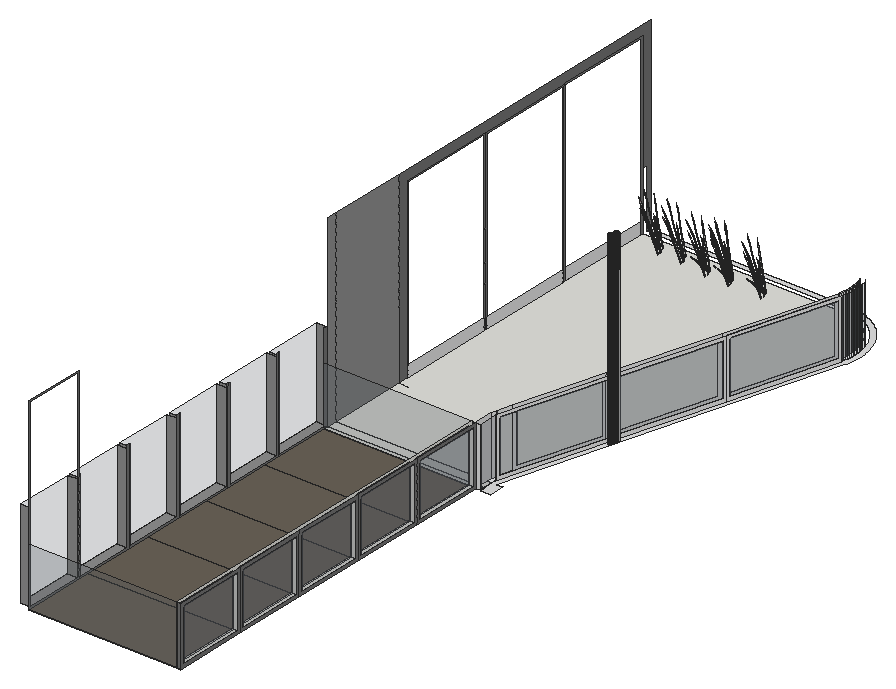
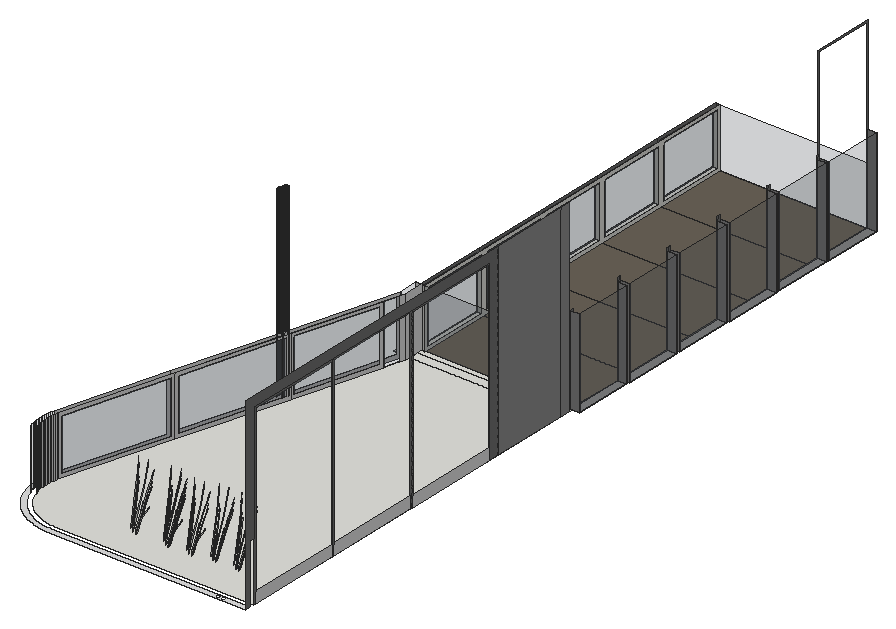
# SketchUp Ruby script. Lengths in inches.
U = 1.inch
M = Sketchup.active_model
def pt(a) = Geom::Point3d.new(a.map { |v| v * U })
def face(e, loops, mat)
  f = e.add_face(loops[0].map { |a| pt(a) })
  loops[1..].each { |l| e.add_face(l.map { |a| pt(a) }).erase! }
  f.material = f.back_material = mat if mat
  f
end
# faces: each face lists its corners as indices into pts; further lists are holes
def faces(e, pts, list, mat = nil) = list.each { |f| face(e, (f[0].is_a?(Array) ? f : [f]).map { |l| l.map { |i| pts[i] } }, mat) }
# xy, xz, yz: faces in a plane at the given z, y or x. An outline is a flat list of corners, or four numbers for a rectangle; further outlines are holes
def ring(l) = l.size == 4 ? [[l[0], l[1]], [l[2], l[1]], [l[2], l[3]], [l[0], l[3]]] : l.each_slice(2).to_a
def flat(e, list, mat, &to3) = list.each { |f| face(e, (f[0].is_a?(Array) ? f : [f]).map { |l| ring(l).map { |u, v| to3.(u, v) } }, mat) }
def xy(e, z, list, mat = nil) = flat(e, list, mat) { |x, y| [x, y, z] }
def xz(e, y, list, mat = nil) = flat(e, list, mat) { |x, z| [x, y, z] }
def yz(e, x, list, mat = nil) = flat(e, list, mat) { |y, z| [x, y, z] }
def lines(e, pts, list) = list.each { |a, b| e.add_line(pt(pts[a]), pt(pts[b])) }
# prism: a flat outline (further loops are holes) pulled along v
def prism(e, loops, v, mat = nil)
  f = face(e, loops, mat); d = Geom::Vector3d.new(v.map { |x| x * U })
  f.pushpull(f.normal.samedirection?(d) ? d.length : -d.length)
end
def box(e, o, s, mat = nil) = prism(e, [[o, [o[0] + s[0], o[1], o[2]], [o[0] + s[0], o[1] + s[1], o[2]], [o[0], o[1] + s[1], o[2]]]], [0, 0, s[2]], mat)
def at(x, y, z, deg = 0) = Geom::Transformation.translation(pt([x, y, z])) * Geom::Transformation.rotation(ORIGIN, Z_AXIS, deg.degrees)
def axes(o, x, y, z) = Geom::Transformation.new([*x, 0, *y, 0, *z, 0, *pt(o).to_a, 1])
def part(name) = M.definitions.add(name)
# library, detail: a bought-in or finely detailed component or shape, given as its bounding box
def library(name, o, s) = part(name).tap { |d| box(d.entities, o, s) }
def detail(e, o, s) = box(e.add_group.entities, o, s)
def put(e, d, t, mat = nil) = e.add_instance(d, t).tap { |i| i.material = mat if mat }
def group(e, t, mat = nil) = e.add_group.tap { |g| g.transformation = t; g.material = mat if mat }.entities
root = M.entities
M.materials.add("Glass_Basic_01").color = [105, 113, 122]
M.materials["Glass_Basic_01"].alpha = 0.25
M.materials.add("LightPink_Translucent").color = [144, 107, 117]
M.materials["LightPink_Translucent"].alpha = 0.75
M.materials.add("M01_Silver_Fog").color = [224, 224, 224]
M.materials.add("M04_Stone_Frost").color = [142, 142, 142]
M.materials.add("M06_Steel_Smoke").color = [114, 114, 114]
M.materials.add("Plaster_04_1K").color = [106, 98, 87]
c1 = part("blade")
p = [[2.15,0.21,22],[0,0.17,0],[0.09,0.45,0],[2.18,0.31,22],[2.29,0.31,22],[0.38,0.45,0],
  [2.48,0.24,33],[2.49,0.24,33],[2.48,0.22,33]]
faces(c1.entities,p,[[0,1,2,3],[4,5,2,3],[6,3,4,7],[8,0,3,6]])
c2 = part("seeds")
p = [[0.3,-0.1,1.38],[-0.01,-0.03,1.59],[-0.01,-0.03,0.03],[0.14,-0.07,-0.07],[0.29,-0.03,3],[0.15,0.01,3.11]]
faces(c2.entities,p,[[0,1,2,3],[1,0,4,5]],"LightPink_Translucent")
c3 = part("blade with seeds")
put(c3.entities,c1,at(0,0,0))
put(c3.entities,c2,axes([2.4,0.25,30.99],[1.5799,-0.05474,1.17369],[-0.12525,1.92788,0.29478],[-0.07173,-0.02425,1.56792]))
xy(root,648,[[210,231,302.38,234],[302.38,231,305.51,234],[305.51,231,306,234],[210,234,302.38,240],[302.38,234,305.51,240],
  [210,240,302.38,240,302.38,243,303.26,246,306,255.36,321.22,307.35,340.07,371.78,359.17,437.01,359.4,437.91,359.63,439,359.83,440.1,359.98,441.21,360.09,442.32,360.16,443.43,360.1875,444.55,360.17,445.67,360.11,446.78,360.01,447.89,359.87,449,359.68,450.1,359.45,451.2,359.18,452.28,358.875,453.35,358.52,454.41,358.13,455.46,357.7,456.49,357.23,457.5,356.73,458.5,356.18,459.47,355.6,460.43,354.98,461.36,354.33,462.26,353.64,463.14,352.92,464,352.17,464.83,351.39,465.62,350.58,466.39,349.74,467.125,348.87,467.83,347.97,468.5,347.05,469.13,346.11,469.73,345.15,470.29,344.16,470.82,343.16,471.3,342.13,471.75,341.09,472.16,340.04,472.53,338.97,472.86,337.89,473.15,336.8,473.4,335.71,473.6,334.6,473.77,333.49,473.89,332.38,473.97,331.45,474,210,474]])
xy(root,648,[[[306,231,312,231,312,240,307.76,240,364.95,435.42,365.24,436.52,365.52,437.84,365.76,439.16,365.94,440.5,366.07,441.84,366.16,443.18,366.1875,444.52,366.17,445.87,366.1,447.21,365.98,448.55,365.8,449.89,365.58,451.21,365.3,452.53,364.98,453.84,364.61,455.13,364.18,456.41,363.71,457.67,363.2,458.91,362.63,460.13,362.02,461.33,361.36,462.5,360.69,463.59,360.66,463.65,359.92,464.77,359.13,465.86,358.3,466.92,357.4375,467.95,357.39,468,356.53,468.95,355.59,469.91,354.61,470.83,353.6,471.72,352.55,472.5625,351.47,473.37,350.37,474.13,349.23,474.85,348.07,475.53,346.88,476.16,345.67,476.75,344.44,477.29,343.1875,477.79,341.92,478.23,340.63,478.63,339.33,478.98,338.02,479.28,336.7,479.52,335.37,479.72,334.03,479.87,332.69,479.96,331.55,480,210,480,210,477,331.5,477,332.53,476.97,333.76,476.88,334.99,476.74,336.2,476.5625,337.41,476.34,338.61,476.0625,339.8,475.75,340.98,475.38,342.14,474.97,343.29,474.52,344.41,474.03,345.52,473.49,346.61,472.91,347.67,472.29,348.71,471.63,349.72,470.93,350.71,470.19,351.67,469.42,352.59,468.61,353.49,467.76,354.35,466.89,355.17,465.98,355.18,465.98,355.97,465.03,356.73,464.0625,357.45,463.0625,358.13,462.04,358.13,462.03,358.77,460.99,359.37,459.91,359.93,458.82,360.45,457.7,360.92,456.5625,361.35,455.41,361.74,454.24,362.08,453.06,362.38,451.86,362.63,450.66,362.83,449.44,362.99,448.22,363.1,447,363.17,445.77,363.1875,444.54,363.16,443.31,363.08,442.08,362.96,440.85,362.79,439.63,362.58,438.42,362.32,437.22,362.06,436.22,343.2,371.78,324.34,307.35,305.51,243,305.51,234,306,234],[228.34,477.03,228.25,477.04,228.17,477.06,228.08,477.08,228,477.11,227.91,477.14,227.84,477.18,227.76,477.22,227.68,477.27,227.54,477.37,227.48,477.43,227.42,477.5,227.36,477.56,227.3125,477.64,227.26,477.71,227.18,477.87,227.15,477.95,227.125,478.03,227.1,478.12,227.09,478.2,227.07,478.29,227.07,478.55,227.08,478.64,227.1,478.73,227.12,478.8125,227.15,478.9,227.18,478.98,227.22,479.06,227.26,479.13,227.31,479.21,227.41,479.35,227.47,479.41,227.61,479.53,227.75,479.63,227.91,479.71,228.07,479.77,228.16,479.79,228.24,479.81,228.33,479.82,228.42,479.82,228.51,479.83,228.59,479.82,228.68,479.81,228.77,479.79,228.85,479.77,228.9375,479.74,229.02,479.71,229.1,479.68,229.18,479.63,229.25,479.59,229.32,479.53,229.39,479.48,229.45,479.42,229.51,479.35,229.57,479.29,229.62,479.22,229.67,479.14,229.71,479.07,229.75,478.99,229.78,478.9,229.81,478.82,229.83,478.74,229.85,478.65,229.86,478.5625,229.87,478.47,229.87,478.39,229.85,478.21,229.83,478.125,229.8125,478.04,229.79,477.96,229.75,477.875,229.72,477.79,229.67,477.72,229.63,477.64,229.58,477.57,229.52,477.5,229.46,477.4375,229.4,477.38,229.33,477.32,229.26,477.27,229.18,477.22,229.11,477.18,229.03,477.14,228.95,477.11,228.86,477.08,228.78,477.06,228.69,477.04,228.6,477.03],[225.03,477.03,224.94,477.04,224.85,477.06,224.77,477.08,224.68,477.11,224.6,477.14,224.52,477.18,224.45,477.22,224.37,477.27,224.23,477.37,224.17,477.43,224.11,477.5,224.05,477.56,224,477.64,223.95,477.71,223.87,477.87,223.84,477.95,223.8125,478.03,223.77,478.2,223.76,478.29,223.76,478.55,223.77,478.64,223.79,478.73,223.81,478.8125,223.84,478.9,223.87,478.98,223.91,479.06,223.95,479.13,223.99,479.21,224.05,479.28,224.1,479.35,224.16,479.41,224.23,479.47,224.29,479.53,224.36,479.58,224.4375,479.63,224.52,479.67,224.6,479.71,224.76,479.77,224.85,479.79,224.93,479.81,225.02,479.82,225.11,479.82,225.19,479.83,225.37,479.81,225.46,479.79,225.54,479.77,225.71,479.71,225.79,479.68,225.86,479.63,225.9375,479.59,226.01,479.53,226.08,479.48,226.14,479.42,226.2,479.35,226.26,479.29,226.3125,479.22,226.36,479.14,226.4,479.07,226.4375,478.99,226.47,478.9,226.5,478.82,226.52,478.74,226.54,478.65,226.55,478.5625,226.55,478.3,226.54,478.21,226.5,478.04,226.47,477.96,226.44,477.875,226.4,477.79,226.36,477.72,226.32,477.64,226.26,477.57,226.21,477.5,226.15,477.4375,226.08,477.38,226.02,477.32,225.95,477.27,225.87,477.22,225.71,477.14,225.55,477.08,225.46,477.06,225.38,477.04,225.29,477.03],[325.27,304.17,325.18,304.18,325.09,304.1875,325.01,304.2,324.92,304.23,324.84,304.25,324.6,304.37,324.39,304.52,324.32,304.58,324.26,304.65,324.11,304.86,324.03,305.02,324,305.1,323.97,305.1875,323.95,305.27,323.9375,305.36,323.93,305.44,323.92,305.53,323.92,305.62,323.93,305.71,323.9375,305.8,323.96,305.88,323.98,305.97,324,306.05,324.12,306.29,324.27,306.5,324.33,306.56,324.4,306.625,324.47,306.68,324.61,306.78,324.77,306.86,324.85,306.89,324.9375,306.92,325.02,306.9375,325.11,306.95,325.2,306.96,325.28,306.97,325.37,306.97,325.55,306.95,325.63,306.93,325.72,306.91,325.88,306.85,325.96,306.8125,326.04,306.77,326.18,306.67,326.25,306.61,326.31,306.55,326.375,306.49,326.43,306.42,326.53,306.28,326.61,306.12,326.64,306.04,326.67,305.95,326.6875,305.87,326.7,305.78,326.71,305.69,326.72,305.61,326.72,305.52,326.7,305.34,326.68,305.26,326.66,305.17,326.6,305.01,326.5625,304.93,326.52,304.85,326.42,304.71,326.3,304.57,326.24,304.51,326.03,304.36,325.87,304.28,325.79,304.25,325.7,304.22,325.62,304.2,325.53,304.1875,325.44,304.17],[326.2,307.35,326.02,307.37,325.9375,307.38,325.85,307.41,325.77,307.43,325.6875,307.47,325.61,307.5,325.53,307.55,325.32,307.7,325.26,307.76,325.14,307.9,325.04,308.04,324.96,308.2,324.93,308.28,324.9,308.37,324.88,308.45,324.87,308.54,324.85,308.71,324.85,308.8,324.87,308.98,324.89,309.0625,324.91,309.15,324.9375,309.23,324.97,309.3125,325.01,309.39,325.05,309.47,325.2,309.68,325.27,309.74,325.33,309.8,325.4,309.86,325.54,309.96,325.7,310.04,325.78,310.07,325.87,310.1,325.95,310.12,326.04,310.13,326.21,310.15,326.3,310.15,326.48,310.13,326.5625,310.11,326.65,310.09,326.73,310.0625,326.8125,310.03,326.89,309.99,326.97,309.95,327.11,309.85,327.25,309.73,327.31,309.67,327.46,309.46,327.54,309.3,327.57,309.22,327.6,309.13,327.62,309.05,327.63,308.96,327.65,308.79,327.65,308.7,327.63,308.52,327.61,308.4375,327.59,308.35,327.56,308.27,327.53,308.1875,327.49,308.11,327.45,308.03,327.4,307.96,327.35,307.88,327.3,307.82,327.17,307.69,326.96,307.54,326.8,307.46,326.72,307.43,326.63,307.4,326.55,307.38,326.46,307.36,326.375,307.35]]],"M01_Silver_Fog")
xy(root,648,[[300,6,303,51],[300,51,303,96],[300,96,303,141],[300,141,303,186],[300,186,303,231]],"M06_Steel_Smoke")
xy(root,648,[[210,6,300,51],[210,51,300,96],[210,96,300,141],[210,141,300,186],[210,186,300,231]],"Plaster_04_1K")
xy(root,649,[[204,7,210,43],[204,45,210,81],[204,83,210,119],[204,121,210,157],[204,159,210,195],
  [204,197,210,233]],"M04_Stone_Frost")
xy(root,650,[[300,8,303,49],[300,53,303,94],[300,98,303,139],[300,143,303,184],[300,188,303,229]])
xz(root,6,[[210,648,300,684]],"Glass_Basic_01")
xz(root,6,[[300,648,303,684]],"M06_Steel_Smoke")
xz(root,7,[[204,649,210,703]],"M04_Stone_Frost")
xz(root,8,[[300,650,303,682]])
xz(root,43,[[204,649,210,703]],"M04_Stone_Frost")
xz(root,45,[[204,649,210,703]],"M04_Stone_Frost")
xz(root,49,[[300,650,303,682]])
xz(root,53,[[300,650,303,682]])
xz(root,81,[[204,649,210,703]],"M04_Stone_Frost")
xz(root,83,[[204,649,210,703]],"M04_Stone_Frost")
xz(root,94,[[300,650,303,682]])
xz(root,98,[[300,650,303,682]])
xz(root,119,[[204,649,210,703]],"M04_Stone_Frost")
xz(root,121,[[204,649,210,703]],"M04_Stone_Frost")
xz(root,139,[[300,650,303,682]])
xz(root,143,[[300,650,303,682]])
xz(root,157,[[204,649,210,703]],"M04_Stone_Frost")
xz(root,159,[[204,649,210,703]],"M04_Stone_Frost")
xz(root,184,[[300,650,303,682]])
xz(root,188,[[300,650,303,682]])
xz(root,195,[[204,649,210,703]],"M04_Stone_Frost")
xz(root,197,[[204,649,210,703]],"M04_Stone_Frost")
xz(root,229,[[300,650,303,682]])
xz(root,231,[[300,648,302.38,684]])
xz(root,231,[[210,648,300,684]],"Glass_Basic_01")
xz(root,231,[[302.38,648,303,684],[303,648,305.51,684]],"M01_Silver_Fog")
xz(root,233,[[204,649,210,703]],"M04_Stone_Frost")
xz(root,304.17,[[325.27,648,325.36,762],[325.36,648,325.44,762]],"M01_Silver_Fog")
xz(root,306.97,[[325.28,648,325.37,762]],"M01_Silver_Fog")
xz(root,307.35,[[326.2,648,326.29,762],[326.29,648,326.375,762]],"M01_Silver_Fog")
xz(root,310.15,[[326.21,648,326.3,762]],"M01_Silver_Fog")
yz(root,204,[[7,649,43,703],[45,649,81,703],[83,649,119,703],[121,649,157,703],[159,649,195,703],
  [197,649,233,703]],"Glass_Basic_01")
yz(root,210,[[295,648,353,655],[355,648,413,655],[415,648,473,655]],"M01_Silver_Fog")
yz(root,210,[[234,648,240,762],[240,648,288,762]],"M04_Stone_Frost")
yz(root,210,[[6,648,44,648,44,705,43,705,43,649,7,649,7,761,43,761,43,705,44,705,44,762,6,762],[44,648,82,648,82,705,81,705,81,649,45,649,45,705,44,705],[82,648,120,648,120,705,119,705,119,649,83,649,83,705,82,705],[120,648,158,648,158,705,157,705,157,649,121,649,121,705,120,705],[158,648,196,648,196,705,195,705,195,649,159,649,159,705,158,705],
  [196,648,231,648,231,649,197,649,197,705,196,705],[288,648,294,648,294,756,474,756,474,684,477,684,477,648,480,648,480,762,288,762],[294,648,295,648,295,755,353,755,353,648,354,648,354,756,294,756],[354,648,355,648,355,755,413,755,413,648,414,648,414,756,354,756],[414,648,415,648,415,755,473,755,473,648,474,648,474,756,414,756],
  [231,649,233,703]],"M06_Steel_Smoke")
yz(root,300,[[[6,648,231,684],[8,650,49,682],[143,650,184,682],[188,650,229,682],[53,650,94,682],[98,650,139,682]]])
yz(root,300,[[8,650,49,682],[53,650,94,682],[98,650,139,682],[143,650,184,682],[188,650,229,682]],"Glass_Basic_01")
yz(root,302.38,[[231,648,243,684]],"M01_Silver_Fog")
yz(root,303,[[8,650,49,682],[53,650,94,682],[98,650,139,682],[143,650,184,682],[188,650,229,682]],"Glass_Basic_01")
yz(root,303,[[[6,648,51,684],[8,650,49,682]],[[51,648,96,684],[53,650,94,682]],[[96,648,141,684],[98,650,139,682]],[[141,648,186,684],[143,650,184,682]],[[186,648,231,684],[188,650,229,682]]],"M06_Steel_Smoke")
yz(root,305.51,[[231,648,243,684]],"Glass_Basic_01")
yz(root,323.92,[[305.53,648,305.62,762]],"M01_Silver_Fog")
yz(root,324.85,[[308.71,648,308.8,762]],"M01_Silver_Fog")
yz(root,326.72,[[305.52,648,305.61,762]],"M01_Silver_Fog")
yz(root,327.65,[[308.7,648,308.79,762]],"M01_Silver_Fog")
p = [[302.38,243,684],[303.26,246,684],[303.26,246,648],[302.38,243,648],[305.51,243,648],[324.34,307.35,648],
  [324.34,307.35,684],[305.51,243,684],[323.78,305.43,682],[323.78,305.43,650],[306.07,244.92,650],[306.07,244.92,682],
  [306,255.36,684],[306,255.36,648],[321.22,307.35,684],[321.22,307.35,648],[320.65,305.43,682],[306.5625,257.28,682],
  [306.5625,257.28,650],[320.65,305.43,650],[324.84,304.25,648],[324.92,304.23,648],[324.92,304.23,762],[324.84,304.25,762],
  [325.01,304.2,648],[325.01,304.2,762],[325.09,304.1875,648],[325.09,304.1875,762],[325.18,304.18,648],[325.18,304.18,762],
  [325.27,304.17,648],[325.27,304.17,762],[325.44,304.17,648],[325.53,304.1875,648],[325.53,304.1875,762],[325.44,304.17,762],
  [325.62,304.2,648],[325.62,304.2,762],[325.7,304.22,648],[325.7,304.22,762],[325.79,304.25,648],[325.79,304.25,762],
  [325.87,304.28,648],[325.87,304.28,762],[324.6,304.37,648],[324.68,304.33,648],[324.68,304.33,762],[324.6,304.37,762],
  [324.76,304.29,648],[324.76,304.29,762],[325.95,304.32,648],[325.95,304.32,762],[326.03,304.36,648],[326.03,304.36,762],
  [324.53,304.42,648],[324.53,304.42,762],[324.46,304.47,648],[324.46,304.47,762],[326.1,304.41,648],[326.1,304.41,762],
  [326.17,304.46,648],[326.17,304.46,762],[324.32,304.58,648],[324.39,304.52,648],[324.39,304.52,762],[324.32,304.58,762],
  [326.24,304.51,648],[326.24,304.51,762],[326.3,304.57,648],[326.3,304.57,762],[324.21,304.72,648],[324.26,304.65,648],
  [324.26,304.65,762],[324.21,304.72,762],[326.36,304.64,648],[326.36,304.64,762],[326.42,304.71,648],[326.42,304.71,762],
  [324.16,304.79,648],[324.16,304.79,762],[326.47,304.78,648],[326.47,304.78,762],[324.11,304.86,648],[324.11,304.86,762],
  [326.52,304.85,648],[326.52,304.85,762],[324.03,305.02,648],[324.07,304.94,648],[324.07,304.94,762],[324.03,305.02,762],
  [326.5625,304.93,648],[326.5625,304.93,762],[326.6,305.01,648],[326.6,305.01,762],[324,305.1,648],[324,305.1,762],
  [326.63,305.09,648],[326.63,305.09,762],[323.97,305.1875,648],[323.97,305.1875,762],[326.66,305.17,648],[326.66,305.17,762],
  [323.95,305.27,648],[323.95,305.27,762],[326.68,305.26,648],[326.68,305.26,762],[323.9375,305.36,648],[323.9375,305.36,762],
  [326.7,305.34,648],[326.7,305.34,762],[326.71,305.43,648],[326.71,305.43,762],[323.93,305.44,648],[323.93,305.44,762],
  [323.92,305.53,648],[323.92,305.53,762],[326.72,305.52,648],[326.72,305.52,762],[323.93,305.71,648],[323.92,305.62,648],
  [323.92,305.62,762],[323.93,305.71,762],[326.72,305.61,648],[326.71,305.69,648],[326.71,305.69,762],[326.72,305.61,762],
  [323.9375,305.8,648],[323.9375,305.8,762],[326.7,305.78,648],[326.7,305.78,762],[323.96,305.88,648],[323.96,305.88,762],
  [326.6875,305.87,648],[326.6875,305.87,762],[323.98,305.97,648],[323.98,305.97,762],[326.67,305.95,648],[326.67,305.95,762],
  [324,306.05,648],[324,306.05,762],[326.64,306.04,648],[326.64,306.04,762],[326.61,306.12,648],[326.61,306.12,762],
  [324.04,306.13,648],[324.04,306.13,762],[324.08,306.21,648],[324.08,306.21,762],[326.57,306.2,648],[326.57,306.2,762],
  [324.12,306.29,648],[324.12,306.29,762],[326.53,306.28,648],[326.53,306.28,762],[324.17,306.36,648],[324.17,306.36,762],
  [326.48,306.35,648],[326.48,306.35,762],[324.22,306.43,648],[324.22,306.43,762],[324.27,306.5,648],[324.27,306.5,762],
  [326.43,306.42,648],[326.43,306.42,762],[326.375,306.49,648],[326.375,306.49,762],[324.33,306.56,648],[324.33,306.56,762],
  [326.31,306.55,648],[326.31,306.55,762],[324.4,306.625,648],[324.4,306.625,762],[324.47,306.68,648],[324.47,306.68,762],
  [326.25,306.61,648],[326.18,306.67,648],[326.18,306.67,762],[326.25,306.61,762],[324.54,306.73,648],[324.54,306.73,762],
  [324.61,306.78,648],[324.61,306.78,762],[326.11,306.72,648],[326.04,306.77,648],[326.04,306.77,762],[326.11,306.72,762],
  [324.69,306.82,648],[324.69,306.82,762],[324.77,306.86,648],[324.77,306.86,762],[325.96,306.8125,648],[325.88,306.85,648],
  [325.88,306.85,762],[325.96,306.8125,762],[324.85,306.89,648],[324.85,306.89,762],[324.9375,306.92,648],[324.9375,306.92,762],
  [325.02,306.9375,648],[325.02,306.9375,762],[325.11,306.95,648],[325.11,306.95,762],[325.63,306.93,648],[325.55,306.95,648],
  [325.55,306.95,762],[325.63,306.93,762],[325.72,306.91,648],[325.72,306.91,762],[325.8,306.88,648],[325.8,306.88,762],
  [325.2,306.96,648],[325.2,306.96,762],[325.28,306.97,648],[325.28,306.97,762],[325.46,306.96,648],[325.37,306.97,648],
  [325.37,306.97,762],[325.46,306.96,762],[340.07,371.78,684],[340.07,371.78,648],[339.51,369.86,650],[339.51,369.86,682],
  [321.78,309.27,682],[321.78,309.27,650],[343.2,371.78,684],[343.2,371.78,648],[324.9,309.27,650],[324.9,309.27,682],
  [342.64,369.86,682],[342.64,369.86,650],[326.11,307.36,648],[326.2,307.35,648],[326.2,307.35,762],[326.11,307.36,762],
  [325.6875,307.47,648],[325.77,307.43,648],[325.77,307.43,762],[325.6875,307.47,762],[325.85,307.41,648],[325.85,307.41,762],
  [325.9375,307.38,648],[326.02,307.37,648],[326.02,307.37,762],[325.9375,307.38,762],[326.375,307.35,648],[326.46,307.36,648],
  [326.46,307.36,762],[326.375,307.35,762],[326.55,307.38,648],[326.55,307.38,762],[326.63,307.4,648],[326.63,307.4,762],
  [326.72,307.43,648],[326.72,307.43,762],[326.8,307.46,648],[326.8,307.46,762],[325.53,307.55,648],[325.61,307.5,648],
  [325.61,307.5,762],[325.53,307.55,762],[325.46,307.6,648],[325.46,307.6,762],[326.88,307.5,648],[326.88,307.5,762],
  [326.96,307.54,648],[326.96,307.54,762],[327.03,307.59,648],[327.03,307.59,762],[325.32,307.7,648],[325.39,307.65,648],
  [325.39,307.65,762],[325.32,307.7,762],[327.1,307.64,648],[327.1,307.64,762],[327.17,307.69,648],[327.17,307.69,762],
  [325.26,307.76,648],[325.26,307.76,762],[327.23,307.75,648],[327.23,307.75,762],[325.14,307.9,648],[325.2,307.83,648],
  [325.2,307.83,762],[325.14,307.9,762],[327.3,307.82,648],[327.3,307.82,762],[327.35,307.88,648],[327.35,307.88,762],
  [325.09,307.97,648],[325.09,307.97,762],[327.4,307.96,648],[327.4,307.96,762],[325.04,308.04,648],[325.04,308.04,762],
  [325,308.12,648],[325,308.12,762],[327.45,308.03,648],[327.45,308.03,762],[327.49,308.11,648],[327.49,308.11,762],
  [324.96,308.2,648],[324.96,308.2,762],[327.53,308.1875,648],[327.53,308.1875,762],[324.93,308.28,648],[324.93,308.28,762],
  [327.56,308.27,648],[327.56,308.27,762],[324.9,308.37,648],[324.9,308.37,762],[327.59,308.35,648],[327.59,308.35,762],
  [324.88,308.45,648],[324.88,308.45,762],[327.61,308.4375,648],[327.61,308.4375,762],[327.63,308.52,648],[327.63,308.52,762],
  [324.87,308.54,648],[324.87,308.54,762],[324.86,308.625,648],[324.86,308.625,762],[327.64,308.61,648],[327.64,308.61,762],
  [324.85,308.71,648],[324.85,308.71,762],[327.65,308.7,648],[327.65,308.7,762],[324.86,308.89,648],[324.85,308.8,648],
  [324.85,308.8,762],[324.86,308.89,762],[327.65,308.79,648],[327.64,308.875,648],[327.64,308.875,762],[327.65,308.79,762],
  [324.87,308.98,648],[324.87,308.98,762],[327.63,308.96,648],[327.63,308.96,762],[324.89,309.0625,648],[324.89,309.0625,762],
  [327.62,309.05,648],[327.62,309.05,762],[327.6,309.13,648],[327.6,309.13,762],[324.91,309.15,648],[324.91,309.15,762],
  [324.9375,309.23,648],[324.9375,309.23,762],[327.57,309.22,648],[327.57,309.22,762],[324.97,309.3125,648],[324.97,309.3125,762],
  [327.54,309.3,648],[327.54,309.3,762],[325.01,309.39,648],[325.01,309.39,762],[327.5,309.38,648],[327.5,309.38,762],
  [325.05,309.47,648],[325.05,309.47,762],[327.46,309.46,648],[327.46,309.46,762],[325.1,309.54,648],[325.1,309.54,762],
  [325.15,309.61,648],[325.15,309.61,762],[327.41,309.53,648],[327.41,309.53,762],[327.36,309.6,648],[327.36,309.6,762],
  [325.2,309.68,648],[325.2,309.68,762],[327.31,309.67,648],[327.31,309.67,762],[325.27,309.74,648],[325.27,309.74,762],
  [325.33,309.8,648],[325.33,309.8,762],[327.25,309.73,648],[327.25,309.73,762],[327.18,309.79,648],[327.18,309.79,762],
  [325.4,309.86,648],[325.4,309.86,762],[327.11,309.85,648],[327.11,309.85,762],[325.47,309.91,648],[325.47,309.91,762],
  [325.54,309.96,648],[325.54,309.96,762],[327.04,309.9,648],[327.04,309.9,762],[326.97,309.95,648],[326.97,309.95,762],
  [325.62,310,648],[325.62,310,762],[325.7,310.04,648],[325.7,310.04,762],[325.78,310.07,648],[325.78,310.07,762],
  [326.8125,310.03,648],[326.73,310.0625,648],[326.73,310.0625,762],[326.8125,310.03,762],[326.89,309.99,648],[326.89,309.99,762],
  [325.87,310.1,648],[325.87,310.1,762],[325.95,310.12,648],[325.95,310.12,762],[326.04,310.13,648],[326.04,310.13,762],
  [326.125,310.14,648],[326.125,310.14,762],[326.21,310.15,648],[326.21,310.15,762],[326.39,310.14,648],[326.3,310.15,648],
  [326.3,310.15,762],[326.39,310.14,762],[326.48,310.13,648],[326.48,310.13,762],[326.5625,310.11,648],[326.5625,310.11,762],
  [326.65,310.09,648],[326.65,310.09,762],[359.17,437.01,648],[359.17,437.01,684],[340.64,373.7,650],[358.6,435.09,650],
  [358.6,435.09,682],[340.64,373.7,682],[362.06,436.22,684],[362.06,436.22,648],[343.76,373.7,682],[361.5,434.3,682],
  [361.5,434.3,650],[343.76,373.7,650],[362.32,437.22,648],[362.32,437.22,684],[359.4,437.91,648],[359.4,437.91,684],
  [362.58,438.42,648],[362.58,438.42,684],[359.63,439,648],[359.63,439,684],[362.79,439.63,648],[362.79,439.63,684],
  [359.83,440.1,648],[359.83,440.1,684],[362.96,440.85,648],[362.96,440.85,684],[359.98,441.21,648],[359.98,441.21,684],
  [363.08,442.08,648],[363.08,442.08,684],[360.09,442.32,648],[360.09,442.32,684],[363.16,443.31,648],[363.16,443.31,684],
  [360.16,443.43,648],[360.16,443.43,684],[363.1875,444.54,648],[363.1875,444.54,684],[360.1875,444.55,648],[360.1875,444.55,684],
  [360.17,445.67,648],[360.17,445.67,684],[363.17,445.77,648],[363.17,445.77,684],[360.11,446.78,648],[360.11,446.78,684],
  [363.1,447,648],[363.1,447,684],[360.01,447.89,648],[360.01,447.89,684],[362.99,448.22,648],[362.99,448.22,684],
  [359.87,449,648],[359.87,449,684],[362.83,449.44,648],[362.83,449.44,684],[359.68,450.1,648],[359.68,450.1,684],
  [362.63,450.66,648],[362.63,450.66,684],[359.45,451.2,648],[359.45,451.2,684],[362.38,451.86,648],[362.38,451.86,684],
  [359.18,452.28,648],[359.18,452.28,684],[362.08,453.06,648],[362.08,453.06,684],[358.875,453.35,648],[358.875,453.35,684],
  [361.74,454.24,648],[361.74,454.24,684],[358.52,454.41,648],[358.52,454.41,684],[361.35,455.41,648],[361.35,455.41,684],
  [213,288,648],[213,287.79,648],[210,288,648],[209.78,288,762],[209.78,288,648],[305.48,242.91,648],
  [305.48,242.91,684],[216,287.79,648]]
faces(root,p,[[0,1,2,3],[[4,5,6,7],[8,9,10,11]],[[12,14,15,13],[16,17,18,19]],[20,21,22,23],[21,24,25,22],[24,26,27,25],[26,28,29,27],[28,30,31,29],
  [32,33,34,35],[33,36,37,34],[36,38,39,37],[38,40,41,39],[40,42,43,41],[44,45,46,47],[45,48,49,46],[48,20,23,49],
  [42,50,51,43],[50,52,53,51],[54,44,47,55],[56,54,55,57],[52,58,59,53],[58,60,61,59],[62,63,64,65],[63,56,57,64],
  [60,66,67,61],[66,68,69,67],[70,71,72,73],[71,62,65,72],[68,74,75,69],[74,76,77,75],[78,70,73,79],[76,80,81,77],
  [82,78,79,83],[80,84,85,81],[86,87,88,89],[87,82,83,88],[84,90,91,85],[90,92,93,91],[94,86,89,95],[92,96,97,93],
  [98,94,95,99],[96,100,101,97],[102,98,99,103],[100,104,105,101],[106,102,103,107],[104,108,109,105],[108,110,111,109],[112,106,107,113],
  [114,112,113,115],[110,116,117,111],[118,119,120,121],[122,123,124,125],[126,118,121,127],[123,128,129,124],[130,126,127,131],[128,132,133,129],
  [134,130,131,135],[132,136,137,133],[138,134,135,139],[136,140,141,137],[140,142,143,141],[144,138,139,145],[146,144,145,147],[142,148,149,143],
  [150,146,147,151],[148,152,153,149],[154,150,151,155],[152,156,157,153],[158,154,155,159],[160,158,159,161],[156,162,163,157],[162,164,165,163],
  [166,160,161,167],[164,168,169,165],[170,166,167,171],[172,170,171,173],[174,175,176,177],[168,174,177,169],[178,172,173,179],[180,178,179,181],
  [182,183,184,185],[175,182,185,176],[186,180,181,187],[188,186,187,189],[190,191,192,193],[183,190,193,184],[194,188,189,195],[196,194,195,197],
  [198,196,197,199],[200,198,199,201],[202,203,204,205],[206,202,205,207],[208,206,207,209],[191,208,209,192],[210,200,201,211],[212,210,211,213],
  [214,215,216,217],[203,214,217,204],[[14,218,219,15],[220,221,222,223]],[[224,6,5,225],[226,227,228,229]],[230,231,232,233],[234,235,236,237],[235,238,239,236],[240,241,242,243],
  [238,240,243,239],[241,230,233,242],[244,245,246,247],[245,248,249,246],[248,250,251,249],[250,252,253,251],[252,254,255,253],[256,257,258,259],
  [260,256,259,261],[257,234,237,258],[254,262,263,255],[262,264,265,263],[264,266,267,265],[268,269,270,271],[269,260,261,270],[266,272,273,267],
  [272,274,275,273],[276,268,271,277],[274,278,279,275],[280,281,282,283],[281,276,277,282],[278,284,285,279],[284,286,287,285],[288,280,283,289],
  [286,290,291,287],[292,288,289,293],[294,292,293,295],[290,296,297,291],[296,298,299,297],[300,294,295,301],[298,302,303,299],[304,300,301,305],
  [302,306,307,303],[308,304,305,309],[306,310,311,307],[312,308,309,313],[310,314,315,311],[314,316,317,315],[318,312,313,319],[320,318,319,321],
  [316,322,323,317],[324,320,321,325],[322,326,327,323],[328,329,330,331],[332,333,334,335],[336,328,331,337],[333,338,339,334],[340,336,337,341],
  [338,342,343,339],[342,344,345,343],[346,340,341,347],[348,346,347,349],[344,350,351,345],[352,348,349,353],[350,354,355,351],[356,352,353,357],
  [354,358,359,355],[360,356,357,361],[358,362,363,359],[364,360,361,365],[366,364,365,367],[362,368,369,363],[368,370,371,369],[372,366,367,373],
  [370,374,375,371],[376,372,373,377],[378,376,377,379],[374,380,381,375],[380,382,383,381],[384,378,379,385],[382,386,387,383],[388,384,385,389],
  [390,388,389,391],[386,392,393,387],[392,394,395,393],[396,390,391,397],[398,396,397,399],[400,398,399,401],[402,403,404,405],[406,402,405,407],
  [394,406,407,395],[408,400,401,409],[410,408,409,411],[412,410,411,413],[414,412,413,415],[416,414,415,417],[418,419,420,421],[422,418,421,423],
  [424,422,423,425],[403,426,427,404],[426,424,425,427],[[428,219,218,429],[430,431,432,433]],[[434,224,225,435],[436,437,438,439]],[442,428,429,443],[446,442,443,447],[450,446,447,451],
  [454,450,451,455],[458,454,455,459],[462,458,459,463],[466,462,463,467],[468,466,467,469],[472,468,469,473],[476,472,473,477],[480,476,477,481],
  [484,480,481,485],[488,484,485,489],[492,488,489,493],[496,492,493,497],[500,496,497,501]],"M01_Silver_Fog")
faces(root,p,[[1,12,13,2],[435,440,441,434],[440,444,445,441],[444,448,449,445],[448,452,453,449],[452,456,457,453],[456,460,461,457],[460,464,465,461],
  [464,470,471,465],[470,474,475,471],[474,478,479,475],[478,482,483,479],[482,486,487,483],[486,490,491,487],[490,494,495,491],[494,498,499,495],
  [498,502,503,499],[9,8,11,10],[17,16,19,18],[221,220,223,222],[227,226,229,228],[431,430,433,432],[437,436,439,438]],"Glass_Basic_01")
lines(root,p,[[504,505],[504,506],[507,508],[509,510],[511,505]])
put(root,c3,axes([260.25,458.68,651.875],[0.11485,0.17291,1.71376],[-0.53072,0.14557,0.13857],[-0.11995,-0.27145,0.73262]))
put(root,c3,axes([274.5,458.68,651.875],[0.11485,0.17291,1.71376],[-0.53072,0.14557,0.13857],[-0.11995,-0.27145,0.73262]))
put(root,c3,axes([294.4,458.68,651.875],[0.11485,0.17291,1.71376],[-0.53072,0.14557,0.13857],[-0.11995,-0.27145,0.73262]))
put(root,c3,axes([231.5,458.68,653.875],[0.11485,0.17291,1.71376],[-0.53072,0.14557,0.13857],[-0.11995,-0.27145,0.73262]))
put(root,c3,axes([245.39,458.68,653.875],[0.11485,0.17291,1.71376],[-0.53072,0.14557,0.13857],[-0.11995,-0.27145,0.73262]))
put(root,c3,axes([274.5,458.68,653.875],[0.11485,0.17291,1.71376],[-0.53072,0.14557,0.13857],[-0.11995,-0.27145,0.73262]))
put(root,c3,axes([261.13,457.53,652.72],[-0.07685,-0.07551,1.74944],[-0.51287,0.04787,-0.27667],[-0.08185,-0.1806,0.14031]))
put(root,c3,axes([275.38,457.53,652.72],[-0.07685,-0.07551,1.74944],[-0.51287,0.04787,-0.27667],[-0.08185,-0.1806,0.14031]))
put(root,c3,axes([295.28,457.53,652.72],[-0.07685,-0.07551,1.74944],[-0.51287,0.04787,-0.27667],[-0.08185,-0.1806,0.14031]))
put(root,c3,axes([262.32,458.43,650.59],[-0.14282,0.10901,1.43002],[-0.42773,-0.19079,-0.30754],[0.07929,-0.23728,0.61141]))
put(root,c3,axes([276.57,458.43,650.59],[-0.14282,0.10901,1.43002],[-0.42773,-0.19079,-0.30754],[0.07929,-0.23728,0.61141]))
put(root,c3,axes([296.47,458.43,650.59],[-0.14282,0.10901,1.43002],[-0.42773,-0.19079,-0.30754],[0.07929,-0.23728,0.61141]))
put(root,c3,axes([233.57,458.43,652.59],[-0.14282,0.10901,1.43002],[-0.42773,-0.19079,-0.30754],[0.07929,-0.23728,0.61141]))
put(root,c3,axes([247.46,458.43,652.59],[-0.14282,0.10901,1.43002],[-0.42773,-0.19079,-0.30754],[0.07929,-0.23728,0.61141]))
put(root,c3,axes([276.57,458.43,652.59],[-0.14282,0.10901,1.43002],[-0.42773,-0.19079,-0.30754],[0.07929,-0.23728,0.61141]))
put(root,c3,axes([261.67,458.81,652.98],[-0.23981,-0.43789,-0.71045],[0.49365,-0.24404,0.08574],[-0.05608,-0.21158,1.00501]))
put(root,c3,axes([275.92,458.81,652.98],[-0.23981,-0.43789,-0.71045],[0.49365,-0.24404,0.08574],[-0.05608,-0.21158,1.00501]))
put(root,c3,axes([295.8125,458.81,652.98],[-0.23981,-0.43789,-0.71045],[0.49365,-0.24404,0.08574],[-0.05608,-0.21158,1.00501]))
put(root,c3,axes([232.92,458.81,654.98],[-0.23981,-0.43789,-0.71045],[0.49365,-0.24404,0.08574],[-0.05608,-0.21158,1.00501]))
put(root,c3,axes([246.81,458.81,654.98],[-0.23981,-0.43789,-0.71045],[0.49365,-0.24404,0.08574],[-0.05608,-0.21158,1.00501]))
put(root,c3,axes([275.92,458.81,654.98],[-0.23981,-0.43789,-0.71045],[0.49365,-0.24404,0.08574],[-0.05608,-0.21158,1.00501]))
put(root,c3,axes([260.11,458.22,650.59],[-0.03043,0.17617,1.43002],[-0.4448,0.14748,-0.30754],[-0.10397,-0.22771,0.61141]))
put(root,c3,axes([274.36,458.22,650.59],[-0.03043,0.17617,1.43002],[-0.4448,0.14748,-0.30754],[-0.10397,-0.22771,0.61141]))
put(root,c3,axes([294.25,458.22,650.59],[-0.03043,0.17617,1.43002],[-0.4448,0.14748,-0.30754],[-0.10397,-0.22771,0.61141]))
put(root,c3,axes([231.36,458.22,652.59],[-0.03043,0.17617,1.43002],[-0.4448,0.14748,-0.30754],[-0.10397,-0.22771,0.61141]))
put(root,c3,axes([245.25,458.22,652.59],[-0.03043,0.17617,1.43002],[-0.4448,0.14748,-0.30754],[-0.10397,-0.22771,0.61141]))
put(root,c3,axes([274.36,458.22,652.59],[-0.03043,0.17617,1.43002],[-0.4448,0.14748,-0.30754],[-0.10397,-0.22771,0.61141]))
put(root,c3,axes([261.25,457.83,649.49],[-0.08428,0.0194,1.76342],[-0.46606,-0.21841,-0.26939],[0.00782,-0.18218,0.30037]))
put(root,c3,axes([275.51,457.83,649.49],[-0.08428,0.0194,1.76342],[-0.46606,-0.21841,-0.26939],[0.00782,-0.18218,0.30037]))
put(root,c3,axes([295.4,457.83,649.49],[-0.08428,0.0194,1.76342],[-0.46606,-0.21841,-0.26939],[0.00782,-0.18218,0.30037]))
put(root,c3,axes([232.51,457.83,651.49],[-0.08428,0.0194,1.76342],[-0.46606,-0.21841,-0.26939],[0.00782,-0.18218,0.30037]))
put(root,c3,axes([246.39,457.83,651.49],[-0.08428,0.0194,1.76342],[-0.46606,-0.21841,-0.26939],[0.00782,-0.18218,0.30037]))
put(root,c3,axes([275.51,457.83,651.49],[-0.08428,0.0194,1.76342],[-0.46606,-0.21841,-0.26939],[0.00782,-0.18218,0.30037]))
put(root,c3,axes([262.66,459.23,652.98],[0.01307,-0.49815,-0.71045],[0.55054,0.03346,0.08574],[0.0581,-0.21104,1.00501]))
put(root,c3,axes([276.92,459.23,652.98],[0.01307,-0.49815,-0.71045],[0.55054,0.03346,0.08574],[0.0581,-0.21104,1.00501]))
put(root,c3,axes([296.8125,459.23,652.98],[0.01307,-0.49815,-0.71045],[0.55054,0.03346,0.08574],[0.0581,-0.21104,1.00501]))
put(root,c3,axes([233.92,459.23,654.98],[0.01307,-0.49815,-0.71045],[0.55054,0.03346,0.08574],[0.0581,-0.21104,1.00501]))
put(root,c3,axes([247.8,459.23,654.98],[0.01307,-0.49815,-0.71045],[0.55054,0.03346,0.08574],[0.0581,-0.21104,1.00501]))
put(root,c3,axes([276.92,459.23,654.98],[0.01307,-0.49815,-0.71045],[0.55054,0.03346,0.08574],[0.0581,-0.21104,1.00501]))
put(root,c3,axes([263.43,458.46,652.72],[-0.00485,-0.10718,1.74944],[-0.40965,-0.30977,-0.27667],[0.06333,-0.18778,0.14031]))
put(root,c3,axes([277.68,458.46,652.72],[-0.00485,-0.10718,1.74944],[-0.40965,-0.30977,-0.27667],[0.06333,-0.18778,0.14031]))
put(root,c3,axes([297.58,458.46,652.72],[-0.00485,-0.10718,1.74944],[-0.40965,-0.30977,-0.27667],[0.06333,-0.18778,0.14031]))
